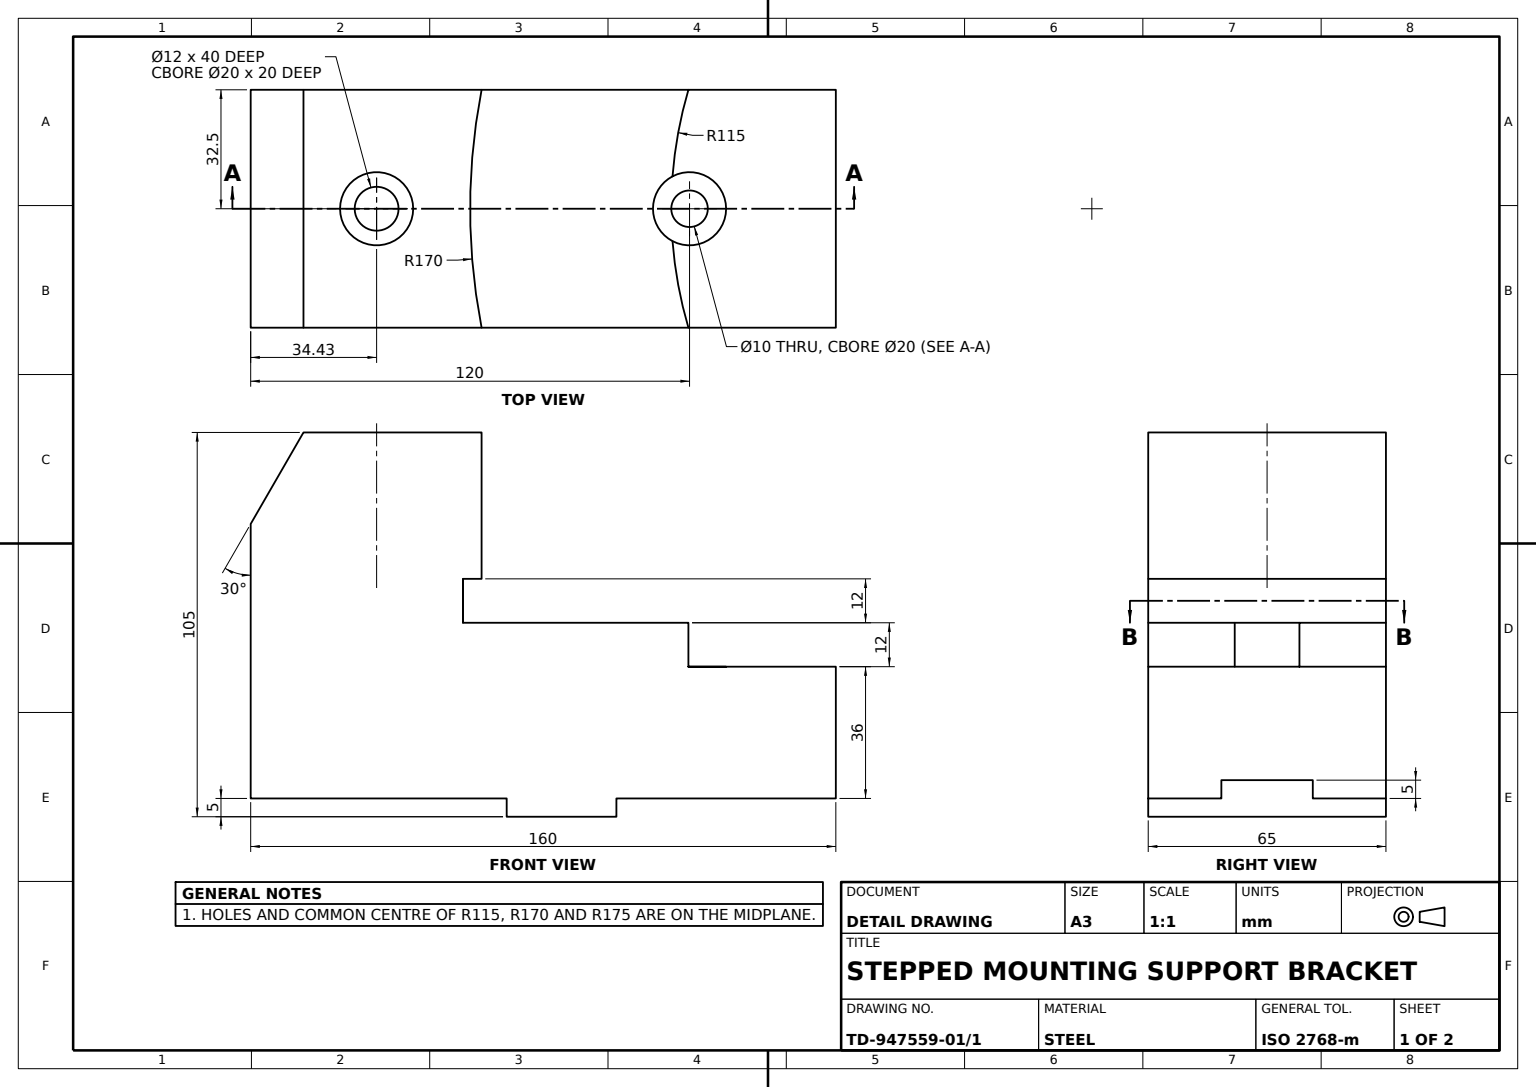
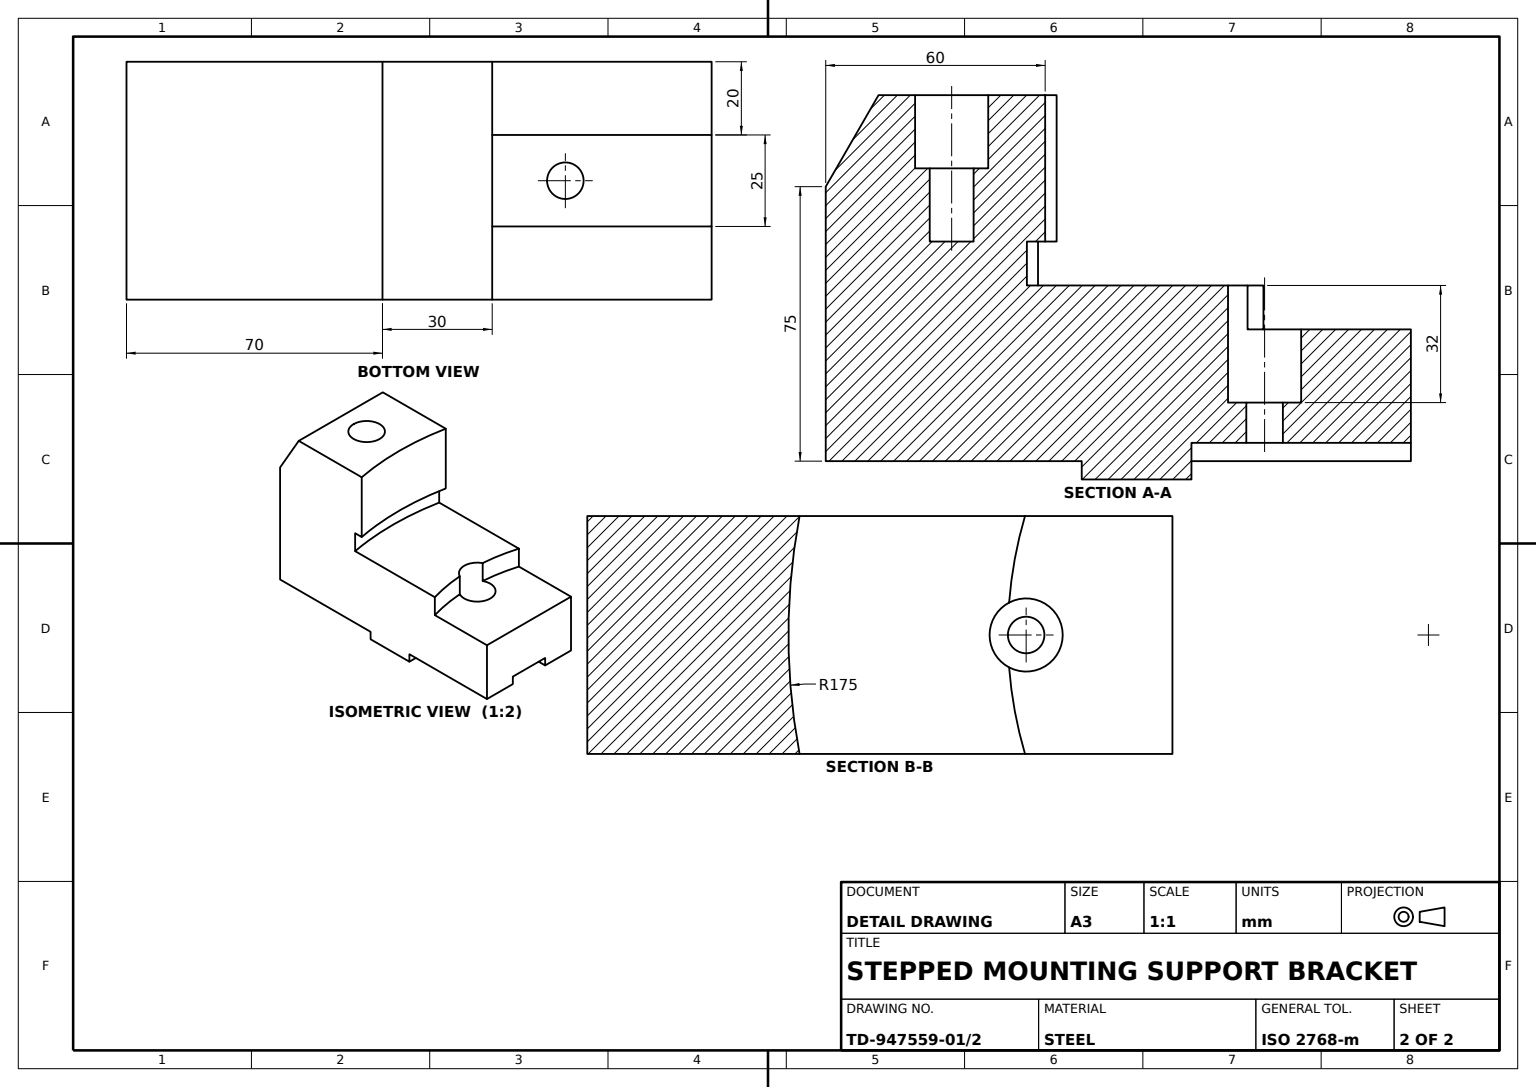
ISO-10303-21;
HEADER;
FILE_DESCRIPTION((''),'2;1');
FILE_NAME('','',(''),(''),'','','');
FILE_SCHEMA(('AUTOMOTIVE_DESIGN'));
ENDSEC;
DATA;
#1=APPLICATION_CONTEXT('');
#2=PRODUCT_CONTEXT('',#1,'mechanical');
#3=PRODUCT('','','',(#2));
#4=PRODUCT_DEFINITION_FORMATION('','',#3);
#5=PRODUCT_DEFINITION_CONTEXT('',#1,'design');
#6=PRODUCT_DEFINITION('','',#4,#5);
#7=PRODUCT_DEFINITION_SHAPE('','',#6);
#8=(LENGTH_UNIT()NAMED_UNIT(*)SI_UNIT(.MILLI.,.METRE.));
#9=(NAMED_UNIT(*)PLANE_ANGLE_UNIT()SI_UNIT($,.RADIAN.));
#10=(NAMED_UNIT(*)SI_UNIT($,.STERADIAN.)SOLID_ANGLE_UNIT());
#11=UNCERTAINTY_MEASURE_WITH_UNIT(LENGTH_MEASURE(0.005),#8,'distance_accuracy_value','');
#12=(GEOMETRIC_REPRESENTATION_CONTEXT(3)GLOBAL_UNCERTAINTY_ASSIGNED_CONTEXT((#11))GLOBAL_UNIT_ASSIGNED_CONTEXT((#8,#9,#10))REPRESENTATION_CONTEXT('',''));
#13=CARTESIAN_POINT('',(-135.566243,0.,80.));
#14=VERTEX_POINT('',#13);
#15=CARTESIAN_POINT('',(-125.566243,0.,80.));
#16=DIRECTION('',(0.,0.,-1.));
#17=DIRECTION('',(-1.,0.,0.));
#18=AXIS2_PLACEMENT_3D('',#15,#16,#17);
#19=CIRCLE('',#18,10.);
#20=EDGE_CURVE('',#14,#14,#19,.F.);
#21=ORIENTED_EDGE('',*,*,#20,.F.);
#22=EDGE_LOOP('',(#21));
#23=FACE_BOUND('',#22,.T.);
#24=CARTESIAN_POINT('',(-135.566243,0.,100.));
#25=VERTEX_POINT('',#24);
#26=CARTESIAN_POINT('',(-125.566243,0.,100.));
#27=AXIS2_PLACEMENT_3D('',#26,#16,#17);
#28=CIRCLE('',#27,10.);
#29=EDGE_CURVE('',#25,#25,#28,.T.);
#30=ORIENTED_EDGE('',*,*,#29,.F.);
#31=EDGE_LOOP('',(#30));
#32=FACE_BOUND('',#31,.T.);
#33=CYLINDRICAL_SURFACE('',#27,10.);
#34=ADVANCED_FACE('',(#23,#32),#33,.F.);
#35=CARTESIAN_POINT('',(-101.955663,-32.5,60.));
#36=VERTEX_POINT('',#35);
#37=CARTESIAN_POINT('',(-101.955663,32.5,60.));
#38=VERTEX_POINT('',#37);
#39=CARTESIAN_POINT('',(70.,0.,60.));
#40=DIRECTION('',(0.,0.,1.));
#41=DIRECTION('',(1.,0.,0.));
#42=AXIS2_PLACEMENT_3D('',#39,#40,#41);
#43=CIRCLE('',#42,175.);
#44=EDGE_CURVE('',#36,#38,#43,.F.);
#45=ORIENTED_EDGE('',*,*,#44,.F.);
#46=CARTESIAN_POINT('',(-101.955663,-32.5,48.));
#47=VERTEX_POINT('',#46);
#48=VECTOR('',#16,1000.);
#49=LINE('',#35,#48);
#50=EDGE_CURVE('',#36,#47,#49,.T.);
#51=ORIENTED_EDGE('',*,*,#50,.T.);
#52=CARTESIAN_POINT('',(-101.955663,32.5,48.));
#53=VERTEX_POINT('',#52);
#54=CARTESIAN_POINT('',(70.,0.,48.));
#55=AXIS2_PLACEMENT_3D('',#54,#40,#41);
#56=CIRCLE('',#55,175.);
#57=EDGE_CURVE('',#53,#47,#56,.T.);
#58=ORIENTED_EDGE('',*,*,#57,.F.);
#59=LINE('',#37,#48);
#60=EDGE_CURVE('',#53,#38,#59,.F.);
#61=ORIENTED_EDGE('',*,*,#60,.T.);
#62=EDGE_LOOP('',(#45,#51,#58,#61));
#63=FACE_BOUND('',#62,.T.);
#64=AXIS2_PLACEMENT_3D('',#39,#16,#17);
#65=CYLINDRICAL_SURFACE('',#64,175.);
#66=ADVANCED_FACE('',(#63),#65,.F.);
#67=CARTESIAN_POINT('',(-44.659091,-8.848326,36.));
#68=VERTEX_POINT('',#67);
#69=CARTESIAN_POINT('',(-44.659091,-8.848326,48.));
#70=VERTEX_POINT('',#69);
#71=CARTESIAN_POINT('',(-44.659091,-8.848326,32.005));
#72=LINE('',#71,#48);
#73=EDGE_CURVE('',#68,#70,#72,.F.);
#74=ORIENTED_EDGE('',*,*,#73,.T.);
#75=CARTESIAN_POINT('',(-40.312057,-32.5,48.));
#76=VERTEX_POINT('',#75);
#77=AXIS2_PLACEMENT_3D('',#54,#16,#41);
#78=CIRCLE('',#77,115.);
#79=EDGE_CURVE('',#76,#70,#78,.T.);
#80=ORIENTED_EDGE('',*,*,#79,.F.);
#81=CARTESIAN_POINT('',(-40.312057,-32.5,36.));
#82=VERTEX_POINT('',#81);
#83=LINE('',#75,#48);
#84=EDGE_CURVE('',#76,#82,#83,.T.);
#85=ORIENTED_EDGE('',*,*,#84,.T.);
#86=CARTESIAN_POINT('',(70.,0.,36.));
#87=AXIS2_PLACEMENT_3D('',#86,#16,#41);
#88=CIRCLE('',#87,115.);
#89=EDGE_CURVE('',#82,#68,#88,.T.);
#90=ORIENTED_EDGE('',*,*,#89,.T.);
#91=EDGE_LOOP('',(#74,#80,#85,#90));
#92=FACE_BOUND('',#91,.T.);
#93=AXIS2_PLACEMENT_3D('',#54,#16,#17);
#94=CYLINDRICAL_SURFACE('',#93,115.);
#95=ADVANCED_FACE('',(#92),#94,.F.);
#96=CARTESIAN_POINT('',(-160.,-32.5,0.));
#97=VERTEX_POINT('',#96);
#98=CARTESIAN_POINT('',(-160.,32.5,0.));
#99=VERTEX_POINT('',#98);
#100=DIRECTION('',(0.,-1.,0.));
#101=VECTOR('',#100,1000.);
#102=LINE('',#98,#101);
#103=EDGE_CURVE('',#97,#99,#102,.F.);
#104=ORIENTED_EDGE('',*,*,#103,.T.);
#105=CARTESIAN_POINT('',(-90.,32.5,0.));
#106=VERTEX_POINT('',#105);
#107=VECTOR('',#41,1000.);
#108=LINE('',#98,#107);
#109=EDGE_CURVE('',#106,#99,#108,.F.);
#110=ORIENTED_EDGE('',*,*,#109,.F.);
#111=CARTESIAN_POINT('',(-90.,-32.5,0.));
#112=VERTEX_POINT('',#111);
#113=LINE('',#105,#101);
#114=EDGE_CURVE('',#106,#112,#113,.T.);
#115=ORIENTED_EDGE('',*,*,#114,.T.);
#116=LINE('',#96,#107);
#117=EDGE_CURVE('',#112,#97,#116,.F.);
#118=ORIENTED_EDGE('',*,*,#117,.T.);
#119=EDGE_LOOP('',(#104,#110,#115,#118));
#120=FACE_BOUND('',#119,.T.);
#121=AXIS2_PLACEMENT_3D('',#98,#40,#41);
#122=PLANE('',#121);
#123=ADVANCED_FACE('',(#120),#122,.F.);
#124=CARTESIAN_POINT('',(0.,-12.5,5.));
#125=VERTEX_POINT('',#124);
#126=CARTESIAN_POINT('',(-60.,-12.5,5.));
#127=VERTEX_POINT('',#126);
#128=CARTESIAN_POINT('',(-63.,-12.5,5.));
#129=LINE('',#128,#107);
#130=EDGE_CURVE('',#125,#127,#129,.F.);
#131=ORIENTED_EDGE('',*,*,#130,.F.);
#132=CARTESIAN_POINT('',(0.,-12.5,0.));
#133=VERTEX_POINT('',#132);
#134=CARTESIAN_POINT('',(0.,-12.5,-5.));
#135=VECTOR('',#40,1000.);
#136=LINE('',#134,#135);
#137=EDGE_CURVE('',#133,#125,#136,.T.);
#138=ORIENTED_EDGE('',*,*,#137,.F.);
#139=CARTESIAN_POINT('',(-60.,-12.5,0.));
#140=VERTEX_POINT('',#139);
#141=CARTESIAN_POINT('',(-160.,-12.5,0.));
#142=VECTOR('',#17,1000.);
#143=LINE('',#141,#142);
#144=EDGE_CURVE('',#133,#140,#143,.T.);
#145=ORIENTED_EDGE('',*,*,#144,.T.);
#146=CARTESIAN_POINT('',(-60.,-12.5,-5.));
#147=LINE('',#146,#48);
#148=EDGE_CURVE('',#127,#140,#147,.T.);
#149=ORIENTED_EDGE('',*,*,#148,.F.);
#150=EDGE_LOOP('',(#131,#138,#145,#149));
#151=FACE_BOUND('',#150,.T.);
#152=CARTESIAN_POINT('',(-63.,-12.5,-5.));
#153=DIRECTION('',(0.,1.,0.));
#154=AXIS2_PLACEMENT_3D('',#152,#153,#40);
#155=PLANE('',#154);
#156=ADVANCED_FACE('',(#151),#155,.T.);
#157=CARTESIAN_POINT('',(-44.659091,8.848326,48.));
#158=VERTEX_POINT('',#157);
#159=CARTESIAN_POINT('',(-44.659091,8.848326,36.));
#160=VERTEX_POINT('',#159);
#161=CARTESIAN_POINT('',(-44.659091,8.848326,32.005));
#162=LINE('',#161,#48);
#163=EDGE_CURVE('',#158,#160,#162,.T.);
#164=ORIENTED_EDGE('',*,*,#163,.T.);
#165=CARTESIAN_POINT('',(-40.312057,32.5,36.));
#166=VERTEX_POINT('',#165);
#167=EDGE_CURVE('',#160,#166,#88,.T.);
#168=ORIENTED_EDGE('',*,*,#167,.T.);
#169=CARTESIAN_POINT('',(-40.312057,32.5,48.));
#170=VERTEX_POINT('',#169);
#171=LINE('',#169,#48);
#172=EDGE_CURVE('',#170,#166,#171,.T.);
#173=ORIENTED_EDGE('',*,*,#172,.F.);
#174=EDGE_CURVE('',#158,#170,#78,.T.);
#175=ORIENTED_EDGE('',*,*,#174,.F.);
#176=EDGE_LOOP('',(#164,#168,#173,#175));
#177=FACE_BOUND('',#176,.T.);
#178=ADVANCED_FACE('',(#177),#94,.F.);
#179=CARTESIAN_POINT('',(-131.566243,0.,60.));
#180=VERTEX_POINT('',#179);
#181=CARTESIAN_POINT('',(-125.566243,0.,60.));
#182=AXIS2_PLACEMENT_3D('',#181,#16,#17);
#183=CIRCLE('',#182,6.);
#184=EDGE_CURVE('',#180,#180,#183,.F.);
#185=ORIENTED_EDGE('',*,*,#184,.F.);
#186=EDGE_LOOP('',(#185));
#187=FACE_BOUND('',#186,.T.);
#188=CARTESIAN_POINT('',(-131.566243,0.,80.));
#189=VERTEX_POINT('',#188);
#190=CIRCLE('',#18,6.);
#191=EDGE_CURVE('',#189,#189,#190,.F.);
#192=ORIENTED_EDGE('',*,*,#191,.T.);
#193=EDGE_LOOP('',(#192));
#194=FACE_BOUND('',#193,.T.);
#195=CYLINDRICAL_SURFACE('',#182,6.);
#196=ADVANCED_FACE('',(#187,#194),#195,.F.);
#197=CARTESIAN_POINT('',(-160.,-32.5,48.));
#198=LINE('',#197,#107);
#199=EDGE_CURVE('',#47,#76,#198,.T.);
#200=ORIENTED_EDGE('',*,*,#199,.T.);
#201=ORIENTED_EDGE('',*,*,#79,.T.);
#202=CARTESIAN_POINT('',(-40.,0.,48.));
#203=AXIS2_PLACEMENT_3D('',#202,#40,#41);
#204=CIRCLE('',#203,10.);
#205=EDGE_CURVE('',#158,#70,#204,.T.);
#206=ORIENTED_EDGE('',*,*,#205,.F.);
#207=ORIENTED_EDGE('',*,*,#174,.T.);
#208=CARTESIAN_POINT('',(-160.,32.5,48.));
#209=LINE('',#208,#142);
#210=EDGE_CURVE('',#170,#53,#209,.T.);
#211=ORIENTED_EDGE('',*,*,#210,.T.);
#212=ORIENTED_EDGE('',*,*,#57,.T.);
#213=EDGE_LOOP('',(#200,#201,#206,#207,#211,#212));
#214=FACE_BOUND('',#213,.T.);
#215=PLANE('',#55);
#216=ADVANCED_FACE('',(#214),#215,.T.);
#217=CARTESIAN_POINT('',(-45.,0.,16.));
#218=VERTEX_POINT('',#217);
#219=CARTESIAN_POINT('',(-40.,0.,16.));
#220=AXIS2_PLACEMENT_3D('',#219,#16,#17);
#221=CIRCLE('',#220,5.);
#222=EDGE_CURVE('',#218,#218,#221,.F.);
#223=ORIENTED_EDGE('',*,*,#222,.F.);
#224=EDGE_LOOP('',(#223));
#225=FACE_BOUND('',#224,.T.);
#226=CARTESIAN_POINT('',(-50.,0.,16.));
#227=VERTEX_POINT('',#226);
#228=CIRCLE('',#220,10.);
#229=EDGE_CURVE('',#227,#227,#228,.F.);
#230=ORIENTED_EDGE('',*,*,#229,.T.);
#231=EDGE_LOOP('',(#230));
#232=FACE_BOUND('',#231,.T.);
#233=PLANE('',#220);
#234=ADVANCED_FACE('',(#225,#232),#233,.F.);
#235=CARTESIAN_POINT('',(-90.,-32.5,-5.));
#236=VERTEX_POINT('',#235);
#237=CARTESIAN_POINT('',(-90.,32.5,-5.));
#238=VERTEX_POINT('',#237);
#239=VECTOR('',#153,1000.);
#240=LINE('',#235,#239);
#241=EDGE_CURVE('',#236,#238,#240,.T.);
#242=ORIENTED_EDGE('',*,*,#241,.T.);
#243=CARTESIAN_POINT('',(-60.,32.5,-5.));
#244=VERTEX_POINT('',#243);
#245=LINE('',#243,#142);
#246=EDGE_CURVE('',#244,#238,#245,.T.);
#247=ORIENTED_EDGE('',*,*,#246,.F.);
#248=CARTESIAN_POINT('',(-60.,-32.5,-5.));
#249=VERTEX_POINT('',#248);
#250=LINE('',#248,#239);
#251=EDGE_CURVE('',#249,#244,#250,.T.);
#252=ORIENTED_EDGE('',*,*,#251,.F.);
#253=LINE('',#248,#142);
#254=EDGE_CURVE('',#249,#236,#253,.T.);
#255=ORIENTED_EDGE('',*,*,#254,.T.);
#256=EDGE_LOOP('',(#242,#247,#252,#255));
#257=FACE_BOUND('',#256,.T.);
#258=AXIS2_PLACEMENT_3D('',#248,#16,#17);
#259=PLANE('',#258);
#260=ADVANCED_FACE('',(#257),#259,.T.);
#261=LINE('',#237,#135);
#262=EDGE_CURVE('',#238,#106,#261,.T.);
#263=ORIENTED_EDGE('',*,*,#262,.F.);
#264=ORIENTED_EDGE('',*,*,#241,.F.);
#265=LINE('',#235,#135);
#266=EDGE_CURVE('',#236,#112,#265,.T.);
#267=ORIENTED_EDGE('',*,*,#266,.T.);
#268=ORIENTED_EDGE('',*,*,#114,.F.);
#269=EDGE_LOOP('',(#263,#264,#267,#268));
#270=FACE_BOUND('',#269,.T.);
#271=AXIS2_PLACEMENT_3D('',#235,#17,#40);
#272=PLANE('',#271);
#273=ADVANCED_FACE('',(#270),#272,.T.);
#274=CARTESIAN_POINT('',(0.,12.5,5.));
#275=VERTEX_POINT('',#274);
#276=CARTESIAN_POINT('',(-60.,12.5,5.));
#277=VERTEX_POINT('',#276);
#278=CARTESIAN_POINT('',(-63.,12.5,5.));
#279=LINE('',#278,#107);
#280=EDGE_CURVE('',#275,#277,#279,.F.);
#281=ORIENTED_EDGE('',*,*,#280,.F.);
#282=LINE('',#124,#239);
#283=EDGE_CURVE('',#125,#275,#282,.T.);
#284=ORIENTED_EDGE('',*,*,#283,.F.);
#285=ORIENTED_EDGE('',*,*,#130,.T.);
#286=CARTESIAN_POINT('',(-60.,-32.5,5.));
#287=LINE('',#286,#239);
#288=EDGE_CURVE('',#127,#277,#287,.T.);
#289=ORIENTED_EDGE('',*,*,#288,.T.);
#290=EDGE_LOOP('',(#281,#284,#285,#289));
#291=FACE_BOUND('',#290,.T.);
#292=CARTESIAN_POINT('',(-45.,0.,5.));
#293=VERTEX_POINT('',#292);
#294=CARTESIAN_POINT('',(-40.,0.,5.));
#295=AXIS2_PLACEMENT_3D('',#294,#16,#17);
#296=CIRCLE('',#295,5.);
#297=EDGE_CURVE('',#293,#293,#296,.T.);
#298=ORIENTED_EDGE('',*,*,#297,.F.);
#299=EDGE_LOOP('',(#298));
#300=FACE_BOUND('',#299,.T.);
#301=AXIS2_PLACEMENT_3D('',#128,#16,#17);
#302=PLANE('',#301);
#303=ADVANCED_FACE('',(#291,#300),#302,.T.);
#304=ORIENTED_EDGE('',*,*,#191,.F.);
#305=EDGE_LOOP('',(#304));
#306=FACE_BOUND('',#305,.T.);
#307=ORIENTED_EDGE('',*,*,#20,.T.);
#308=EDGE_LOOP('',(#307));
#309=FACE_BOUND('',#308,.T.);
#310=PLANE('',#18);
#311=ADVANCED_FACE('',(#306,#309),#310,.F.);
#312=CARTESIAN_POINT('',(-60.,12.5,0.));
#313=VERTEX_POINT('',#312);
#314=CARTESIAN_POINT('',(-60.,32.5,0.));
#315=VERTEX_POINT('',#314);
#316=LINE('',#314,#239);
#317=EDGE_CURVE('',#313,#315,#316,.T.);
#318=ORIENTED_EDGE('',*,*,#317,.T.);
#319=CARTESIAN_POINT('',(0.,32.5,0.));
#320=VERTEX_POINT('',#319);
#321=EDGE_CURVE('',#320,#315,#108,.F.);
#322=ORIENTED_EDGE('',*,*,#321,.F.);
#323=CARTESIAN_POINT('',(0.,12.5,0.));
#324=VERTEX_POINT('',#323);
#325=LINE('',#319,#101);
#326=EDGE_CURVE('',#324,#320,#325,.F.);
#327=ORIENTED_EDGE('',*,*,#326,.F.);
#328=CARTESIAN_POINT('',(-160.,12.5,0.));
#329=LINE('',#328,#107);
#330=EDGE_CURVE('',#313,#324,#329,.T.);
#331=ORIENTED_EDGE('',*,*,#330,.F.);
#332=EDGE_LOOP('',(#318,#322,#327,#331));
#333=FACE_BOUND('',#332,.T.);
#334=ADVANCED_FACE('',(#333),#122,.F.);
#335=ORIENTED_EDGE('',*,*,#229,.F.);
#336=EDGE_LOOP('',(#335));
#337=FACE_BOUND('',#336,.T.);
#338=ORIENTED_EDGE('',*,*,#73,.F.);
#339=CARTESIAN_POINT('',(-40.,0.,36.));
#340=AXIS2_PLACEMENT_3D('',#339,#16,#17);
#341=CIRCLE('',#340,10.);
#342=EDGE_CURVE('',#160,#68,#341,.T.);
#343=ORIENTED_EDGE('',*,*,#342,.F.);
#344=ORIENTED_EDGE('',*,*,#163,.F.);
#345=ORIENTED_EDGE('',*,*,#205,.T.);
#346=EDGE_LOOP('',(#338,#343,#344,#345));
#347=FACE_BOUND('',#346,.T.);
#348=CYLINDRICAL_SURFACE('',#340,10.);
#349=ADVANCED_FACE('',(#337,#347),#348,.F.);
#350=ORIENTED_EDGE('',*,*,#184,.T.);
#351=EDGE_LOOP('',(#350));
#352=FACE_BOUND('',#351,.T.);
#353=PLANE('',#182);
#354=ADVANCED_FACE('',(#352),#353,.F.);
#355=CARTESIAN_POINT('',(-60.,32.5,5.));
#356=LINE('',#355,#48);
#357=EDGE_CURVE('',#315,#244,#356,.T.);
#358=ORIENTED_EDGE('',*,*,#357,.T.);
#359=ORIENTED_EDGE('',*,*,#246,.T.);
#360=ORIENTED_EDGE('',*,*,#262,.T.);
#361=ORIENTED_EDGE('',*,*,#109,.T.);
#362=CARTESIAN_POINT('',(-160.,32.5,75.));
#363=VERTEX_POINT('',#362);
#364=CARTESIAN_POINT('',(-160.,32.5,36.));
#365=LINE('',#364,#48);
#366=EDGE_CURVE('',#99,#363,#365,.F.);
#367=ORIENTED_EDGE('',*,*,#366,.T.);
#368=CARTESIAN_POINT('',(-145.566243,32.5,100.));
#369=VERTEX_POINT('',#368);
#370=CARTESIAN_POINT('',(-176.887495,32.5,45.75));
#371=DIRECTION('',(-0.5,0.,-0.866025404));
#372=VECTOR('',#371,1000.);
#373=LINE('',#370,#372);
#374=EDGE_CURVE('',#363,#369,#373,.F.);
#375=ORIENTED_EDGE('',*,*,#374,.T.);
#376=CARTESIAN_POINT('',(-96.864466,32.5,100.));
#377=VERTEX_POINT('',#376);
#378=CARTESIAN_POINT('',(-160.,32.5,100.));
#379=LINE('',#378,#107);
#380=EDGE_CURVE('',#369,#377,#379,.T.);
#381=ORIENTED_EDGE('',*,*,#380,.T.);
#382=CARTESIAN_POINT('',(-96.864466,32.5,60.));
#383=VERTEX_POINT('',#382);
#384=CARTESIAN_POINT('',(-96.864466,32.5,103.));
#385=LINE('',#384,#48);
#386=EDGE_CURVE('',#383,#377,#385,.F.);
#387=ORIENTED_EDGE('',*,*,#386,.F.);
#388=CARTESIAN_POINT('',(-160.,32.5,60.));
#389=LINE('',#388,#142);
#390=EDGE_CURVE('',#383,#38,#389,.T.);
#391=ORIENTED_EDGE('',*,*,#390,.T.);
#392=ORIENTED_EDGE('',*,*,#60,.F.);
#393=ORIENTED_EDGE('',*,*,#210,.F.);
#394=ORIENTED_EDGE('',*,*,#172,.T.);
#395=CARTESIAN_POINT('',(0.,32.5,36.));
#396=VERTEX_POINT('',#395);
#397=LINE('',#364,#107);
#398=EDGE_CURVE('',#396,#166,#397,.F.);
#399=ORIENTED_EDGE('',*,*,#398,.F.);
#400=LINE('',#395,#48);
#401=EDGE_CURVE('',#320,#396,#400,.F.);
#402=ORIENTED_EDGE('',*,*,#401,.F.);
#403=ORIENTED_EDGE('',*,*,#321,.T.);
#404=EDGE_LOOP('',(#358,#359,#360,#361,#367,#375,#381,#387,#391,#392,#393,#394,#399,#402,#403));
#405=FACE_BOUND('',#404,.T.);
#406=AXIS2_PLACEMENT_3D('',#364,#100,#16);
#407=PLANE('',#406);
#408=ADVANCED_FACE('',(#405),#407,.F.);
#409=ORIENTED_EDGE('',*,*,#144,.F.);
#410=CARTESIAN_POINT('',(0.,-32.5,0.));
#411=VERTEX_POINT('',#410);
#412=EDGE_CURVE('',#411,#133,#325,.F.);
#413=ORIENTED_EDGE('',*,*,#412,.F.);
#414=CARTESIAN_POINT('',(-60.,-32.5,0.));
#415=VERTEX_POINT('',#414);
#416=EDGE_CURVE('',#411,#415,#116,.F.);
#417=ORIENTED_EDGE('',*,*,#416,.T.);
#418=EDGE_CURVE('',#415,#140,#316,.T.);
#419=ORIENTED_EDGE('',*,*,#418,.T.);
#420=EDGE_LOOP('',(#409,#413,#417,#419));
#421=FACE_BOUND('',#420,.T.);
#422=ADVANCED_FACE('',(#421),#122,.F.);
#423=ORIENTED_EDGE('',*,*,#390,.F.);
#424=CARTESIAN_POINT('',(-96.864466,-32.5,60.));
#425=VERTEX_POINT('',#424);
#426=CIRCLE('',#42,170.);
#427=EDGE_CURVE('',#383,#425,#426,.T.);
#428=ORIENTED_EDGE('',*,*,#427,.T.);
#429=CARTESIAN_POINT('',(-160.,-32.5,60.));
#430=LINE('',#429,#107);
#431=EDGE_CURVE('',#36,#425,#430,.T.);
#432=ORIENTED_EDGE('',*,*,#431,.F.);
#433=ORIENTED_EDGE('',*,*,#44,.T.);
#434=EDGE_LOOP('',(#423,#428,#432,#433));
#435=FACE_BOUND('',#434,.T.);
#436=PLANE('',#42);
#437=ADVANCED_FACE('',(#435),#436,.F.);
#438=ORIENTED_EDGE('',*,*,#366,.F.);
#439=ORIENTED_EDGE('',*,*,#103,.F.);
#440=CARTESIAN_POINT('',(-160.,-32.5,75.));
#441=VERTEX_POINT('',#440);
#442=LINE('',#96,#135);
#443=EDGE_CURVE('',#441,#97,#442,.F.);
#444=ORIENTED_EDGE('',*,*,#443,.F.);
#445=CARTESIAN_POINT('',(-160.,-56.,75.));
#446=LINE('',#445,#239);
#447=EDGE_CURVE('',#441,#363,#446,.T.);
#448=ORIENTED_EDGE('',*,*,#447,.T.);
#449=EDGE_LOOP('',(#438,#439,#444,#448));
#450=FACE_BOUND('',#449,.T.);
#451=CARTESIAN_POINT('',(-160.,0.,0.));
#452=AXIS2_PLACEMENT_3D('',#451,#17,#40);
#453=PLANE('',#452);
#454=ADVANCED_FACE('',(#450),#453,.T.);
#455=LINE('',#274,#48);
#456=EDGE_CURVE('',#275,#324,#455,.T.);
#457=ORIENTED_EDGE('',*,*,#456,.F.);
#458=ORIENTED_EDGE('',*,*,#280,.T.);
#459=LINE('',#276,#135);
#460=EDGE_CURVE('',#313,#277,#459,.T.);
#461=ORIENTED_EDGE('',*,*,#460,.F.);
#462=ORIENTED_EDGE('',*,*,#330,.T.);
#463=EDGE_LOOP('',(#457,#458,#461,#462));
#464=FACE_BOUND('',#463,.T.);
#465=AXIS2_PLACEMENT_3D('',#278,#100,#16);
#466=PLANE('',#465);
#467=ADVANCED_FACE('',(#464),#466,.T.);
#468=ORIENTED_EDGE('',*,*,#447,.F.);
#469=CARTESIAN_POINT('',(-145.566243,-32.5,100.));
#470=VERTEX_POINT('',#469);
#471=CARTESIAN_POINT('',(-192.475953,-32.5,18.75));
#472=DIRECTION('',(0.5,0.,0.866025404));
#473=VECTOR('',#472,1000.);
#474=LINE('',#471,#473);
#475=EDGE_CURVE('',#470,#441,#474,.F.);
#476=ORIENTED_EDGE('',*,*,#475,.F.);
#477=CARTESIAN_POINT('',(-145.566243,-56.,100.));
#478=LINE('',#477,#239);
#479=EDGE_CURVE('',#470,#369,#478,.T.);
#480=ORIENTED_EDGE('',*,*,#479,.T.);
#481=ORIENTED_EDGE('',*,*,#374,.F.);
#482=EDGE_LOOP('',(#468,#476,#480,#481));
#483=FACE_BOUND('',#482,.T.);
#484=DIRECTION('',(-0.866025404,0.,0.5));
#485=AXIS2_PLACEMENT_3D('',#445,#484,#472);
#486=PLANE('',#485);
#487=ADVANCED_FACE('',(#483),#486,.T.);
#488=CARTESIAN_POINT('',(0.,-32.5,36.));
#489=VERTEX_POINT('',#488);
#490=LINE('',#488,#239);
#491=EDGE_CURVE('',#396,#489,#490,.F.);
#492=ORIENTED_EDGE('',*,*,#491,.F.);
#493=ORIENTED_EDGE('',*,*,#398,.T.);
#494=ORIENTED_EDGE('',*,*,#167,.F.);
#495=ORIENTED_EDGE('',*,*,#342,.T.);
#496=ORIENTED_EDGE('',*,*,#89,.F.);
#497=CARTESIAN_POINT('',(-160.,-32.5,36.));
#498=LINE('',#497,#107);
#499=EDGE_CURVE('',#489,#82,#498,.F.);
#500=ORIENTED_EDGE('',*,*,#499,.F.);
#501=EDGE_LOOP('',(#492,#493,#494,#495,#496,#500));
#502=FACE_BOUND('',#501,.T.);
#503=AXIS2_PLACEMENT_3D('',#497,#16,#17);
#504=PLANE('',#503);
#505=ADVANCED_FACE('',(#502),#504,.F.);
#506=ORIENTED_EDGE('',*,*,#357,.F.);
#507=ORIENTED_EDGE('',*,*,#317,.F.);
#508=ORIENTED_EDGE('',*,*,#460,.T.);
#509=ORIENTED_EDGE('',*,*,#288,.F.);
#510=ORIENTED_EDGE('',*,*,#148,.T.);
#511=ORIENTED_EDGE('',*,*,#418,.F.);
#512=LINE('',#286,#48);
#513=EDGE_CURVE('',#415,#249,#512,.T.);
#514=ORIENTED_EDGE('',*,*,#513,.T.);
#515=ORIENTED_EDGE('',*,*,#251,.T.);
#516=EDGE_LOOP('',(#506,#507,#508,#509,#510,#511,#514,#515));
#517=FACE_BOUND('',#516,.T.);
#518=AXIS2_PLACEMENT_3D('',#286,#41,#16);
#519=PLANE('',#518);
#520=ADVANCED_FACE('',(#517),#519,.T.);
#521=ORIENTED_EDGE('',*,*,#29,.T.);
#522=EDGE_LOOP('',(#521));
#523=FACE_BOUND('',#522,.T.);
#524=ORIENTED_EDGE('',*,*,#479,.F.);
#525=CARTESIAN_POINT('',(-96.864466,-32.5,100.));
#526=VERTEX_POINT('',#525);
#527=CARTESIAN_POINT('',(-93.,-32.5,100.));
#528=LINE('',#527,#142);
#529=EDGE_CURVE('',#526,#470,#528,.T.);
#530=ORIENTED_EDGE('',*,*,#529,.F.);
#531=CARTESIAN_POINT('',(70.,0.,100.));
#532=AXIS2_PLACEMENT_3D('',#531,#16,#17);
#533=CIRCLE('',#532,170.);
#534=EDGE_CURVE('',#377,#526,#533,.F.);
#535=ORIENTED_EDGE('',*,*,#534,.F.);
#536=ORIENTED_EDGE('',*,*,#380,.F.);
#537=EDGE_LOOP('',(#524,#530,#535,#536));
#538=FACE_BOUND('',#537,.T.);
#539=CARTESIAN_POINT('',(0.,0.,100.));
#540=AXIS2_PLACEMENT_3D('',#539,#16,#17);
#541=PLANE('',#540);
#542=ADVANCED_FACE('',(#523,#538),#541,.F.);
#543=ORIENTED_EDGE('',*,*,#412,.T.);
#544=ORIENTED_EDGE('',*,*,#137,.T.);
#545=ORIENTED_EDGE('',*,*,#283,.T.);
#546=ORIENTED_EDGE('',*,*,#456,.T.);
#547=ORIENTED_EDGE('',*,*,#326,.T.);
#548=ORIENTED_EDGE('',*,*,#401,.T.);
#549=ORIENTED_EDGE('',*,*,#491,.T.);
#550=LINE('',#410,#135);
#551=EDGE_CURVE('',#489,#411,#550,.F.);
#552=ORIENTED_EDGE('',*,*,#551,.T.);
#553=EDGE_LOOP('',(#543,#544,#545,#546,#547,#548,#549,#552));
#554=FACE_BOUND('',#553,.T.);
#555=CARTESIAN_POINT('',(0.,0.,0.));
#556=AXIS2_PLACEMENT_3D('',#555,#17,#40);
#557=PLANE('',#556);
#558=ADVANCED_FACE('',(#554),#557,.F.);
#559=ORIENTED_EDGE('',*,*,#222,.T.);
#560=EDGE_LOOP('',(#559));
#561=FACE_BOUND('',#560,.T.);
#562=ORIENTED_EDGE('',*,*,#297,.T.);
#563=EDGE_LOOP('',(#562));
#564=FACE_BOUND('',#563,.T.);
#565=CARTESIAN_POINT('',(-40.,0.,-56.216561));
#566=AXIS2_PLACEMENT_3D('',#565,#16,#17);
#567=CYLINDRICAL_SURFACE('',#566,5.);
#568=ADVANCED_FACE('',(#561,#564),#567,.F.);
#569=ORIENTED_EDGE('',*,*,#427,.F.);
#570=ORIENTED_EDGE('',*,*,#386,.T.);
#571=ORIENTED_EDGE('',*,*,#534,.T.);
#572=CARTESIAN_POINT('',(-96.864466,-32.5,103.));
#573=LINE('',#572,#48);
#574=EDGE_CURVE('',#526,#425,#573,.T.);
#575=ORIENTED_EDGE('',*,*,#574,.T.);
#576=EDGE_LOOP('',(#569,#570,#571,#575));
#577=FACE_BOUND('',#576,.T.);
#578=CARTESIAN_POINT('',(70.,0.,103.));
#579=AXIS2_PLACEMENT_3D('',#578,#16,#17);
#580=CYLINDRICAL_SURFACE('',#579,170.);
#581=ADVANCED_FACE('',(#577),#580,.F.);
#582=ORIENTED_EDGE('',*,*,#551,.F.);
#583=ORIENTED_EDGE('',*,*,#499,.T.);
#584=ORIENTED_EDGE('',*,*,#84,.F.);
#585=ORIENTED_EDGE('',*,*,#199,.F.);
#586=ORIENTED_EDGE('',*,*,#50,.F.);
#587=ORIENTED_EDGE('',*,*,#431,.T.);
#588=ORIENTED_EDGE('',*,*,#574,.F.);
#589=ORIENTED_EDGE('',*,*,#529,.T.);
#590=ORIENTED_EDGE('',*,*,#475,.T.);
#591=ORIENTED_EDGE('',*,*,#443,.T.);
#592=ORIENTED_EDGE('',*,*,#117,.F.);
#593=ORIENTED_EDGE('',*,*,#266,.F.);
#594=ORIENTED_EDGE('',*,*,#254,.F.);
#595=ORIENTED_EDGE('',*,*,#513,.F.);
#596=ORIENTED_EDGE('',*,*,#416,.F.);
#597=EDGE_LOOP('',(#582,#583,#584,#585,#586,#587,#588,#589,#590,#591,#592,#593,#594,#595,#596));
#598=FACE_BOUND('',#597,.T.);
#599=AXIS2_PLACEMENT_3D('',#96,#153,#40);
#600=PLANE('',#599);
#601=ADVANCED_FACE('',(#598),#600,.F.);
#602=CLOSED_SHELL('',(#34,#66,#95,#123,#156,#178,#196,#216,#234,#260,#273,#303,#311,#334,#349,#354,#408,#422,#437,#454,#467,#487,#505,#520,#542,#558,#568,#581,#601));
#603=MANIFOLD_SOLID_BREP('',#602);
#604=ADVANCED_BREP_SHAPE_REPRESENTATION('',(#603),#12);
#605=SHAPE_DEFINITION_REPRESENTATION(#7,#604);
ENDSEC;
END-ISO-10303-21;
